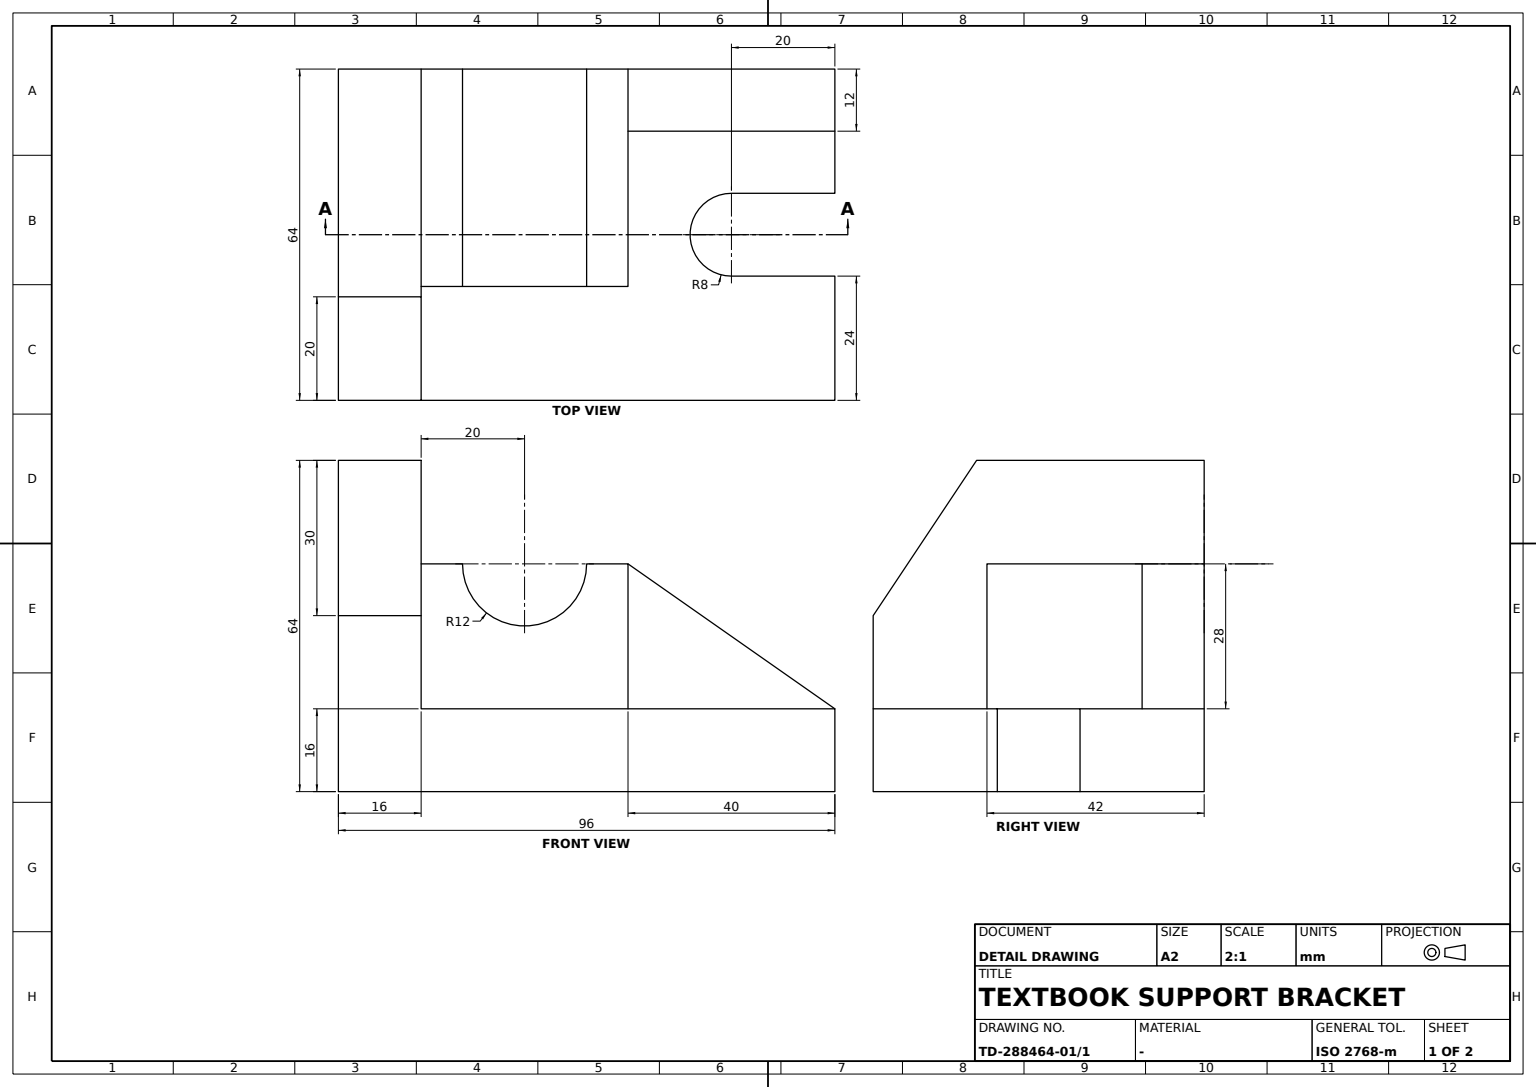
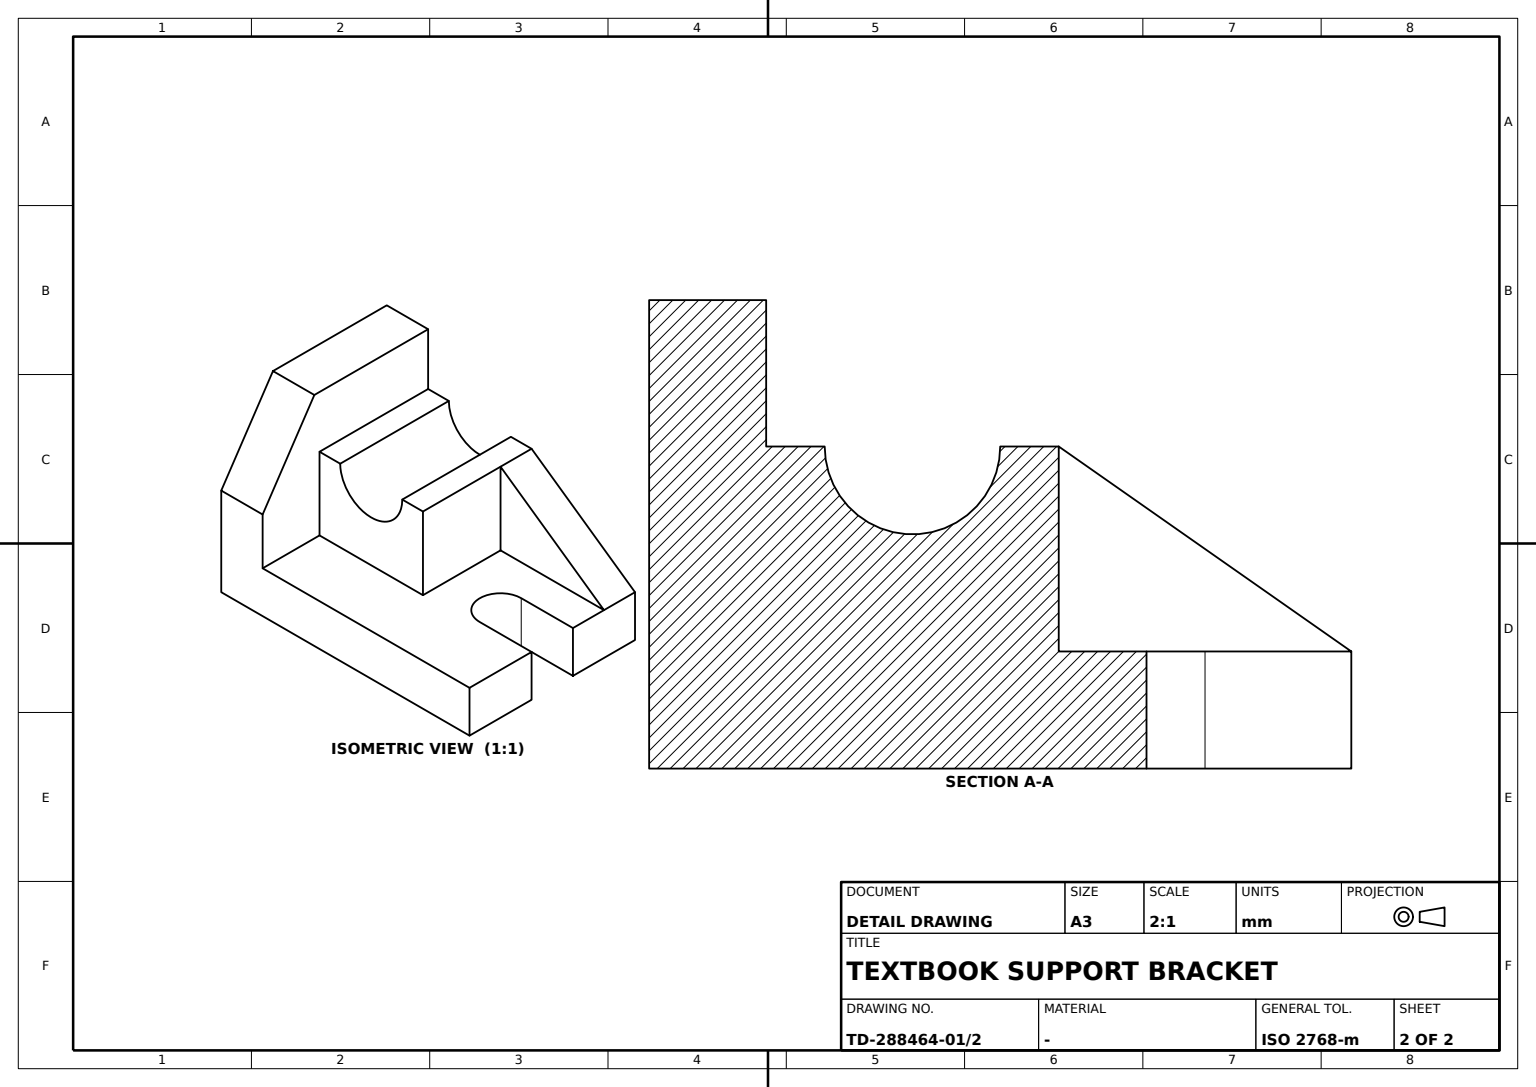
ISO-10303-21;
HEADER;
FILE_DESCRIPTION((''),'2;1');
FILE_NAME('','',(''),(''),'','','');
FILE_SCHEMA(('AUTOMOTIVE_DESIGN'));
ENDSEC;
DATA;
#1=APPLICATION_CONTEXT('');
#2=PRODUCT_CONTEXT('',#1,'mechanical');
#3=PRODUCT('','','',(#2));
#4=PRODUCT_DEFINITION_FORMATION('','',#3);
#5=PRODUCT_DEFINITION_CONTEXT('',#1,'design');
#6=PRODUCT_DEFINITION('','',#4,#5);
#7=PRODUCT_DEFINITION_SHAPE('','',#6);
#8=(LENGTH_UNIT()NAMED_UNIT(*)SI_UNIT(.MILLI.,.METRE.));
#9=(NAMED_UNIT(*)PLANE_ANGLE_UNIT()SI_UNIT($,.RADIAN.));
#10=(NAMED_UNIT(*)SI_UNIT($,.STERADIAN.)SOLID_ANGLE_UNIT());
#11=UNCERTAINTY_MEASURE_WITH_UNIT(LENGTH_MEASURE(0.005),#8,'distance_accuracy_value','');
#12=(GEOMETRIC_REPRESENTATION_CONTEXT(3)GLOBAL_UNCERTAINTY_ASSIGNED_CONTEXT((#11))GLOBAL_UNIT_ASSIGNED_CONTEXT((#8,#9,#10))REPRESENTATION_CONTEXT('',''));
#13=CARTESIAN_POINT('',(-32.,-32.,36.));
#14=VERTEX_POINT('',#13);
#15=CARTESIAN_POINT('',(10.,-32.,36.));
#16=VERTEX_POINT('',#15);
#17=CARTESIAN_POINT('',(0.,-32.,36.));
#18=DIRECTION('',(1.,0.,0.));
#19=VECTOR('',#18,1000.);
#20=LINE('',#17,#19);
#21=EDGE_CURVE('',#14,#16,#20,.T.);
#22=ORIENTED_EDGE('',*,*,#21,.F.);
#23=CARTESIAN_POINT('',(-32.,-32.,56.));
#24=VERTEX_POINT('',#23);
#25=CARTESIAN_POINT('',(-32.,-32.,0.));
#26=DIRECTION('',(0.,0.,1.));
#27=VECTOR('',#26,1000.);
#28=LINE('',#25,#27);
#29=EDGE_CURVE('',#14,#24,#28,.T.);
#30=ORIENTED_EDGE('',*,*,#29,.T.);
#31=CARTESIAN_POINT('',(12.,-32.,56.));
#32=VERTEX_POINT('',#31);
#33=LINE('',#23,#19);
#34=EDGE_CURVE('',#24,#32,#33,.T.);
#35=ORIENTED_EDGE('',*,*,#34,.T.);
#36=CARTESIAN_POINT('',(32.,-32.,26.));
#37=VERTEX_POINT('',#36);
#38=DIRECTION('',(0.554700196,0.,-0.832050294));
#39=VECTOR('',#38,1000.);
#40=LINE('',#31,#39);
#41=EDGE_CURVE('',#32,#37,#40,.T.);
#42=ORIENTED_EDGE('',*,*,#41,.T.);
#43=CARTESIAN_POINT('',(32.,-32.,8.));
#44=VERTEX_POINT('',#43);
#45=CARTESIAN_POINT('',(32.,-32.,0.));
#46=DIRECTION('',(0.,0.,-1.));
#47=VECTOR('',#46,1000.);
#48=LINE('',#45,#47);
#49=EDGE_CURVE('',#37,#44,#48,.T.);
#50=ORIENTED_EDGE('',*,*,#49,.T.);
#51=CARTESIAN_POINT('',(10.,-32.,8.));
#52=VERTEX_POINT('',#51);
#53=CARTESIAN_POINT('',(0.,-32.,8.));
#54=DIRECTION('',(-1.,0.,0.));
#55=VECTOR('',#54,1000.);
#56=LINE('',#53,#55);
#57=EDGE_CURVE('',#44,#52,#56,.T.);
#58=ORIENTED_EDGE('',*,*,#57,.T.);
#59=CARTESIAN_POINT('',(10.,-32.,0.));
#60=LINE('',#59,#27);
#61=EDGE_CURVE('',#52,#16,#60,.T.);
#62=ORIENTED_EDGE('',*,*,#61,.T.);
#63=EDGE_LOOP('',(#22,#30,#35,#42,#50,#58,#62));
#64=FACE_BOUND('',#63,.T.);
#65=CARTESIAN_POINT('',(0.,-32.,0.));
#66=DIRECTION('',(0.,-1.,0.));
#67=AXIS2_PLACEMENT_3D('',#65,#66,#18);
#68=PLANE('',#67);
#69=ADVANCED_FACE('',(#64),#68,.F.);
#70=CARTESIAN_POINT('',(-8.,48.,8.));
#71=VERTEX_POINT('',#70);
#72=CARTESIAN_POINT('',(-8.,48.,-8.));
#73=VERTEX_POINT('',#72);
#74=LINE('',#72,#47);
#75=EDGE_CURVE('',#71,#73,#74,.T.);
#76=ORIENTED_EDGE('',*,*,#75,.F.);
#77=CARTESIAN_POINT('',(-8.,28.,8.));
#78=VERTEX_POINT('',#77);
#79=VECTOR('',#66,1000.);
#80=LINE('',#70,#79);
#81=EDGE_CURVE('',#71,#78,#80,.T.);
#82=ORIENTED_EDGE('',*,*,#81,.T.);
#83=CARTESIAN_POINT('',(-8.,28.,-8.));
#84=VERTEX_POINT('',#83);
#85=LINE('',#83,#27);
#86=EDGE_CURVE('',#78,#84,#85,.F.);
#87=ORIENTED_EDGE('',*,*,#86,.T.);
#88=CARTESIAN_POINT('',(-8.,-48.,-8.));
#89=LINE('',#88,#79);
#90=EDGE_CURVE('',#73,#84,#89,.T.);
#91=ORIENTED_EDGE('',*,*,#90,.F.);
#92=EDGE_LOOP('',(#76,#82,#87,#91));
#93=FACE_BOUND('',#92,.T.);
#94=AXIS2_PLACEMENT_3D('',#70,#18,#66);
#95=PLANE('',#94);
#96=ADVANCED_FACE('',(#93),#95,.T.);
#97=CARTESIAN_POINT('',(-32.,-24.,36.));
#98=VERTEX_POINT('',#97);
#99=CARTESIAN_POINT('',(-32.,0.,36.));
#100=DIRECTION('',(0.,1.,0.));
#101=VECTOR('',#100,1000.);
#102=LINE('',#99,#101);
#103=EDGE_CURVE('',#14,#98,#102,.T.);
#104=ORIENTED_EDGE('',*,*,#103,.F.);
#105=ORIENTED_EDGE('',*,*,#21,.T.);
#106=CARTESIAN_POINT('',(10.,-24.,36.));
#107=VERTEX_POINT('',#106);
#108=LINE('',#15,#101);
#109=EDGE_CURVE('',#16,#107,#108,.T.);
#110=ORIENTED_EDGE('',*,*,#109,.T.);
#111=LINE('',#97,#55);
#112=EDGE_CURVE('',#98,#107,#111,.F.);
#113=ORIENTED_EDGE('',*,*,#112,.F.);
#114=EDGE_LOOP('',(#104,#105,#110,#113));
#115=FACE_BOUND('',#114,.T.);
#116=AXIS2_PLACEMENT_3D('',#13,#46,#100);
#117=PLANE('',#116);
#118=ADVANCED_FACE('',(#115),#117,.F.);
#119=CARTESIAN_POINT('',(-32.,48.,-8.));
#120=VERTEX_POINT('',#119);
#121=CARTESIAN_POINT('',(0.,48.,-8.));
#122=LINE('',#121,#19);
#123=EDGE_CURVE('',#120,#73,#122,.T.);
#124=ORIENTED_EDGE('',*,*,#123,.T.);
#125=ORIENTED_EDGE('',*,*,#90,.T.);
#126=CARTESIAN_POINT('',(8.,28.,-8.));
#127=VERTEX_POINT('',#126);
#128=CARTESIAN_POINT('',(0.,28.,-8.));
#129=AXIS2_PLACEMENT_3D('',#128,#46,#54);
#130=CIRCLE('',#129,8.);
#131=EDGE_CURVE('',#127,#84,#130,.T.);
#132=ORIENTED_EDGE('',*,*,#131,.F.);
#133=CARTESIAN_POINT('',(8.,48.,-8.));
#134=VERTEX_POINT('',#133);
#135=LINE('',#126,#79);
#136=EDGE_CURVE('',#134,#127,#135,.T.);
#137=ORIENTED_EDGE('',*,*,#136,.F.);
#138=CARTESIAN_POINT('',(32.,48.,-8.));
#139=VERTEX_POINT('',#138);
#140=EDGE_CURVE('',#134,#139,#122,.T.);
#141=ORIENTED_EDGE('',*,*,#140,.T.);
#142=CARTESIAN_POINT('',(32.,-48.,-8.));
#143=VERTEX_POINT('',#142);
#144=CARTESIAN_POINT('',(32.,0.,-8.));
#145=LINE('',#144,#101);
#146=EDGE_CURVE('',#143,#139,#145,.T.);
#147=ORIENTED_EDGE('',*,*,#146,.F.);
#148=CARTESIAN_POINT('',(-32.,-48.,-8.));
#149=VERTEX_POINT('',#148);
#150=CARTESIAN_POINT('',(0.,-48.,-8.));
#151=LINE('',#150,#19);
#152=EDGE_CURVE('',#149,#143,#151,.T.);
#153=ORIENTED_EDGE('',*,*,#152,.F.);
#154=CARTESIAN_POINT('',(-32.,0.,-8.));
#155=LINE('',#154,#101);
#156=EDGE_CURVE('',#149,#120,#155,.T.);
#157=ORIENTED_EDGE('',*,*,#156,.T.);
#158=EDGE_LOOP('',(#124,#125,#132,#137,#141,#147,#153,#157));
#159=FACE_BOUND('',#158,.T.);
#160=AXIS2_PLACEMENT_3D('',#150,#46,#100);
#161=PLANE('',#160);
#162=ADVANCED_FACE('',(#159),#161,.T.);
#163=CARTESIAN_POINT('',(-20.,8.,36.));
#164=VERTEX_POINT('',#163);
#165=CARTESIAN_POINT('',(-20.,8.,8.));
#166=VERTEX_POINT('',#165);
#167=LINE('',#163,#47);
#168=EDGE_CURVE('',#164,#166,#167,.T.);
#169=ORIENTED_EDGE('',*,*,#168,.T.);
#170=CARTESIAN_POINT('',(-20.,48.,8.));
#171=VERTEX_POINT('',#170);
#172=LINE('',#170,#79);
#173=EDGE_CURVE('',#171,#166,#172,.T.);
#174=ORIENTED_EDGE('',*,*,#173,.F.);
#175=DIRECTION('',(0.,-0.819231921,0.573462344));
#176=VECTOR('',#175,1000.);
#177=LINE('',#170,#176);
#178=EDGE_CURVE('',#171,#164,#177,.T.);
#179=ORIENTED_EDGE('',*,*,#178,.T.);
#180=EDGE_LOOP('',(#169,#174,#179));
#181=FACE_BOUND('',#180,.T.);
#182=CARTESIAN_POINT('',(-20.,0.,0.));
#183=AXIS2_PLACEMENT_3D('',#182,#54,#66);
#184=PLANE('',#183);
#185=ADVANCED_FACE('',(#181),#184,.F.);
#186=CARTESIAN_POINT('',(-32.,-48.,56.));
#187=VERTEX_POINT('',#186);
#188=LINE('',#186,#101);
#189=EDGE_CURVE('',#187,#24,#188,.T.);
#190=ORIENTED_EDGE('',*,*,#189,.T.);
#191=ORIENTED_EDGE('',*,*,#29,.F.);
#192=ORIENTED_EDGE('',*,*,#103,.T.);
#193=VERTEX_POINT('',#99);
#194=CARTESIAN_POINT('',(-32.,-12.,36.));
#195=AXIS2_PLACEMENT_3D('',#194,#18,#46);
#196=CIRCLE('',#195,12.);
#197=EDGE_CURVE('',#193,#98,#196,.F.);
#198=ORIENTED_EDGE('',*,*,#197,.F.);
#199=CARTESIAN_POINT('',(-32.,8.,36.));
#200=VERTEX_POINT('',#199);
#201=LINE('',#13,#79);
#202=EDGE_CURVE('',#200,#193,#201,.T.);
#203=ORIENTED_EDGE('',*,*,#202,.F.);
#204=CARTESIAN_POINT('',(-32.,48.,8.));
#205=VERTEX_POINT('',#204);
#206=CARTESIAN_POINT('',(-32.,19.543624,27.919463));
#207=LINE('',#206,#176);
#208=EDGE_CURVE('',#205,#200,#207,.T.);
#209=ORIENTED_EDGE('',*,*,#208,.F.);
#210=CARTESIAN_POINT('',(-32.,48.,0.));
#211=LINE('',#210,#27);
#212=EDGE_CURVE('',#120,#205,#211,.T.);
#213=ORIENTED_EDGE('',*,*,#212,.F.);
#214=ORIENTED_EDGE('',*,*,#156,.F.);
#215=CARTESIAN_POINT('',(-32.,-48.,0.));
#216=LINE('',#215,#47);
#217=EDGE_CURVE('',#187,#149,#216,.T.);
#218=ORIENTED_EDGE('',*,*,#217,.F.);
#219=EDGE_LOOP('',(#190,#191,#192,#198,#203,#209,#213,#214,#218));
#220=FACE_BOUND('',#219,.T.);
#221=CARTESIAN_POINT('',(-32.,0.,0.));
#222=AXIS2_PLACEMENT_3D('',#221,#18,#100);
#223=PLANE('',#222);
#224=ADVANCED_FACE('',(#220),#223,.F.);
#225=CARTESIAN_POINT('',(8.,48.,8.));
#226=VERTEX_POINT('',#225);
#227=LINE('',#225,#47);
#228=EDGE_CURVE('',#226,#134,#227,.T.);
#229=ORIENTED_EDGE('',*,*,#228,.T.);
#230=ORIENTED_EDGE('',*,*,#136,.T.);
#231=CARTESIAN_POINT('',(8.,28.,8.));
#232=VERTEX_POINT('',#231);
#233=LINE('',#126,#27);
#234=EDGE_CURVE('',#232,#127,#233,.F.);
#235=ORIENTED_EDGE('',*,*,#234,.F.);
#236=LINE('',#231,#101);
#237=EDGE_CURVE('',#232,#226,#236,.T.);
#238=ORIENTED_EDGE('',*,*,#237,.T.);
#239=EDGE_LOOP('',(#229,#230,#235,#238));
#240=FACE_BOUND('',#239,.T.);
#241=AXIS2_PLACEMENT_3D('',#231,#54,#100);
#242=PLANE('',#241);
#243=ADVANCED_FACE('',(#240),#242,.T.);
#244=ORIENTED_EDGE('',*,*,#217,.T.);
#245=ORIENTED_EDGE('',*,*,#152,.T.);
#246=CARTESIAN_POINT('',(32.,-48.,26.));
#247=VERTEX_POINT('',#246);
#248=CARTESIAN_POINT('',(32.,-48.,0.));
#249=LINE('',#248,#47);
#250=EDGE_CURVE('',#247,#143,#249,.T.);
#251=ORIENTED_EDGE('',*,*,#250,.F.);
#252=CARTESIAN_POINT('',(12.,-48.,56.));
#253=VERTEX_POINT('',#252);
#254=LINE('',#252,#39);
#255=EDGE_CURVE('',#253,#247,#254,.T.);
#256=ORIENTED_EDGE('',*,*,#255,.F.);
#257=LINE('',#186,#19);
#258=EDGE_CURVE('',#187,#253,#257,.T.);
#259=ORIENTED_EDGE('',*,*,#258,.F.);
#260=EDGE_LOOP('',(#244,#245,#251,#256,#259));
#261=FACE_BOUND('',#260,.T.);
#262=CARTESIAN_POINT('',(0.,-48.,8.));
#263=AXIS2_PLACEMENT_3D('',#262,#66,#46);
#264=PLANE('',#263);
#265=ADVANCED_FACE('',(#261),#264,.T.);
#266=ORIENTED_EDGE('',*,*,#75,.T.);
#267=ORIENTED_EDGE('',*,*,#123,.F.);
#268=ORIENTED_EDGE('',*,*,#212,.T.);
#269=CARTESIAN_POINT('',(0.,48.,8.));
#270=LINE('',#269,#19);
#271=EDGE_CURVE('',#205,#171,#270,.T.);
#272=ORIENTED_EDGE('',*,*,#271,.T.);
#273=EDGE_CURVE('',#171,#71,#270,.T.);
#274=ORIENTED_EDGE('',*,*,#273,.T.);
#275=EDGE_LOOP('',(#266,#267,#268,#272,#274));
#276=FACE_BOUND('',#275,.T.);
#277=AXIS2_PLACEMENT_3D('',#121,#100,#26);
#278=PLANE('',#277);
#279=ADVANCED_FACE('',(#276),#278,.T.);
#280=LINE('',#252,#101);
#281=EDGE_CURVE('',#253,#32,#280,.T.);
#282=ORIENTED_EDGE('',*,*,#281,.F.);
#283=ORIENTED_EDGE('',*,*,#255,.T.);
#284=LINE('',#246,#101);
#285=EDGE_CURVE('',#247,#37,#284,.T.);
#286=ORIENTED_EDGE('',*,*,#285,.T.);
#287=ORIENTED_EDGE('',*,*,#41,.F.);
#288=EDGE_LOOP('',(#282,#283,#286,#287));
#289=FACE_BOUND('',#288,.T.);
#290=DIRECTION('',(0.832050294,0.,0.554700196));
#291=AXIS2_PLACEMENT_3D('',#252,#290,#38);
#292=PLANE('',#291);
#293=ADVANCED_FACE('',(#289),#292,.T.);
#294=CARTESIAN_POINT('',(10.,0.,36.));
#295=VERTEX_POINT('',#294);
#296=LINE('',#99,#55);
#297=EDGE_CURVE('',#193,#295,#296,.F.);
#298=ORIENTED_EDGE('',*,*,#297,.T.);
#299=CARTESIAN_POINT('',(10.,8.,36.));
#300=VERTEX_POINT('',#299);
#301=LINE('',#294,#79);
#302=EDGE_CURVE('',#300,#295,#301,.T.);
#303=ORIENTED_EDGE('',*,*,#302,.F.);
#304=LINE('',#199,#19);
#305=EDGE_CURVE('',#164,#300,#304,.T.);
#306=ORIENTED_EDGE('',*,*,#305,.F.);
#307=EDGE_CURVE('',#200,#164,#304,.T.);
#308=ORIENTED_EDGE('',*,*,#307,.F.);
#309=ORIENTED_EDGE('',*,*,#202,.T.);
#310=EDGE_LOOP('',(#298,#303,#306,#308,#309));
#311=FACE_BOUND('',#310,.T.);
#312=ADVANCED_FACE('',(#311),#117,.F.);
#313=ORIENTED_EDGE('',*,*,#86,.F.);
#314=CARTESIAN_POINT('',(0.,28.,8.));
#315=AXIS2_PLACEMENT_3D('',#314,#26,#66);
#316=CIRCLE('',#315,8.);
#317=EDGE_CURVE('',#78,#232,#316,.T.);
#318=ORIENTED_EDGE('',*,*,#317,.T.);
#319=ORIENTED_EDGE('',*,*,#234,.T.);
#320=ORIENTED_EDGE('',*,*,#131,.T.);
#321=EDGE_LOOP('',(#313,#318,#319,#320));
#322=FACE_BOUND('',#321,.T.);
#323=AXIS2_PLACEMENT_3D('',#128,#26,#18);
#324=CYLINDRICAL_SURFACE('',#323,8.);
#325=ADVANCED_FACE('',(#322),#324,.F.);
#326=ORIENTED_EDGE('',*,*,#189,.F.);
#327=ORIENTED_EDGE('',*,*,#258,.T.);
#328=ORIENTED_EDGE('',*,*,#281,.T.);
#329=ORIENTED_EDGE('',*,*,#34,.F.);
#330=EDGE_LOOP('',(#326,#327,#328,#329));
#331=FACE_BOUND('',#330,.T.);
#332=AXIS2_PLACEMENT_3D('',#186,#26,#18);
#333=PLANE('',#332);
#334=ADVANCED_FACE('',(#331),#333,.T.);
#335=CARTESIAN_POINT('',(32.,48.,8.));
#336=VERTEX_POINT('',#335);
#337=CARTESIAN_POINT('',(32.,48.,0.));
#338=LINE('',#337,#27);
#339=EDGE_CURVE('',#139,#336,#338,.T.);
#340=ORIENTED_EDGE('',*,*,#339,.F.);
#341=ORIENTED_EDGE('',*,*,#140,.F.);
#342=ORIENTED_EDGE('',*,*,#228,.F.);
#343=EDGE_CURVE('',#226,#336,#270,.T.);
#344=ORIENTED_EDGE('',*,*,#343,.T.);
#345=EDGE_LOOP('',(#340,#341,#342,#344));
#346=FACE_BOUND('',#345,.T.);
#347=ADVANCED_FACE('',(#346),#278,.T.);
#348=CARTESIAN_POINT('',(10.,-12.,36.));
#349=AXIS2_PLACEMENT_3D('',#348,#54,#26);
#350=CIRCLE('',#349,12.);
#351=EDGE_CURVE('',#295,#107,#350,.T.);
#352=ORIENTED_EDGE('',*,*,#351,.T.);
#353=ORIENTED_EDGE('',*,*,#109,.F.);
#354=ORIENTED_EDGE('',*,*,#61,.F.);
#355=CARTESIAN_POINT('',(10.,8.,8.));
#356=VERTEX_POINT('',#355);
#357=CARTESIAN_POINT('',(10.,48.,8.));
#358=LINE('',#357,#79);
#359=EDGE_CURVE('',#356,#52,#358,.T.);
#360=ORIENTED_EDGE('',*,*,#359,.F.);
#361=LINE('',#299,#47);
#362=EDGE_CURVE('',#300,#356,#361,.T.);
#363=ORIENTED_EDGE('',*,*,#362,.F.);
#364=ORIENTED_EDGE('',*,*,#302,.T.);
#365=EDGE_LOOP('',(#352,#353,#354,#360,#363,#364));
#366=FACE_BOUND('',#365,.T.);
#367=CARTESIAN_POINT('',(10.,0.,0.));
#368=AXIS2_PLACEMENT_3D('',#367,#54,#66);
#369=PLANE('',#368);
#370=ADVANCED_FACE('',(#366),#369,.F.);
#371=ORIENTED_EDGE('',*,*,#57,.F.);
#372=CARTESIAN_POINT('',(32.,0.,8.));
#373=LINE('',#372,#79);
#374=EDGE_CURVE('',#336,#44,#373,.T.);
#375=ORIENTED_EDGE('',*,*,#374,.F.);
#376=ORIENTED_EDGE('',*,*,#343,.F.);
#377=ORIENTED_EDGE('',*,*,#237,.F.);
#378=ORIENTED_EDGE('',*,*,#317,.F.);
#379=ORIENTED_EDGE('',*,*,#81,.F.);
#380=ORIENTED_EDGE('',*,*,#273,.F.);
#381=ORIENTED_EDGE('',*,*,#173,.T.);
#382=CARTESIAN_POINT('',(0.,8.,8.));
#383=LINE('',#382,#19);
#384=EDGE_CURVE('',#166,#356,#383,.T.);
#385=ORIENTED_EDGE('',*,*,#384,.T.);
#386=ORIENTED_EDGE('',*,*,#359,.T.);
#387=EDGE_LOOP('',(#371,#375,#376,#377,#378,#379,#380,#381,#385,#386));
#388=FACE_BOUND('',#387,.T.);
#389=AXIS2_PLACEMENT_3D('',#269,#26,#66);
#390=PLANE('',#389);
#391=ADVANCED_FACE('',(#388),#390,.T.);
#392=ORIENTED_EDGE('',*,*,#49,.F.);
#393=ORIENTED_EDGE('',*,*,#285,.F.);
#394=ORIENTED_EDGE('',*,*,#250,.T.);
#395=ORIENTED_EDGE('',*,*,#146,.T.);
#396=ORIENTED_EDGE('',*,*,#339,.T.);
#397=ORIENTED_EDGE('',*,*,#374,.T.);
#398=EDGE_LOOP('',(#392,#393,#394,#395,#396,#397));
#399=FACE_BOUND('',#398,.T.);
#400=CARTESIAN_POINT('',(32.,0.,0.));
#401=AXIS2_PLACEMENT_3D('',#400,#18,#100);
#402=PLANE('',#401);
#403=ADVANCED_FACE('',(#399),#402,.T.);
#404=ORIENTED_EDGE('',*,*,#178,.F.);
#405=ORIENTED_EDGE('',*,*,#271,.F.);
#406=ORIENTED_EDGE('',*,*,#208,.T.);
#407=ORIENTED_EDGE('',*,*,#307,.T.);
#408=EDGE_LOOP('',(#404,#405,#406,#407));
#409=FACE_BOUND('',#408,.T.);
#410=DIRECTION('',(0.,0.573462344,0.819231921));
#411=AXIS2_PLACEMENT_3D('',#204,#410,#175);
#412=PLANE('',#411);
#413=ADVANCED_FACE('',(#409),#412,.T.);
#414=ORIENTED_EDGE('',*,*,#362,.T.);
#415=ORIENTED_EDGE('',*,*,#384,.F.);
#416=ORIENTED_EDGE('',*,*,#168,.F.);
#417=ORIENTED_EDGE('',*,*,#305,.T.);
#418=EDGE_LOOP('',(#414,#415,#416,#417));
#419=FACE_BOUND('',#418,.T.);
#420=AXIS2_PLACEMENT_3D('',#199,#66,#46);
#421=PLANE('',#420);
#422=ADVANCED_FACE('',(#419),#421,.F.);
#423=ORIENTED_EDGE('',*,*,#112,.T.);
#424=ORIENTED_EDGE('',*,*,#351,.F.);
#425=ORIENTED_EDGE('',*,*,#297,.F.);
#426=ORIENTED_EDGE('',*,*,#197,.T.);
#427=EDGE_LOOP('',(#423,#424,#425,#426));
#428=FACE_BOUND('',#427,.T.);
#429=CARTESIAN_POINT('',(-11.,-12.,36.));
#430=AXIS2_PLACEMENT_3D('',#429,#54,#66);
#431=CYLINDRICAL_SURFACE('',#430,12.);
#432=ADVANCED_FACE('',(#428),#431,.F.);
#433=CLOSED_SHELL('',(#69,#96,#118,#162,#185,#224,#243,#265,#279,#293,#312,#325,#334,#347,#370,#391,#403,#413,#422,#432));
#434=MANIFOLD_SOLID_BREP('',#433);
#435=ADVANCED_BREP_SHAPE_REPRESENTATION('',(#434),#12);
#436=SHAPE_DEFINITION_REPRESENTATION(#7,#435);
ENDSEC;
END-ISO-10303-21;
